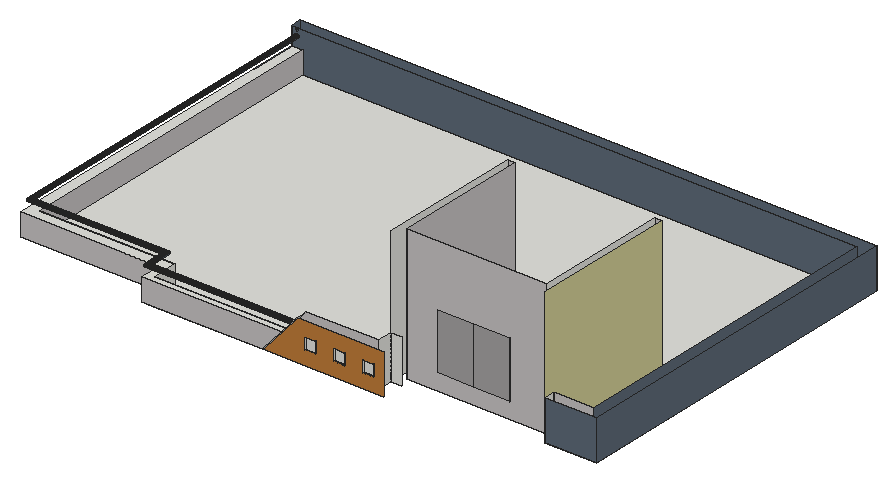
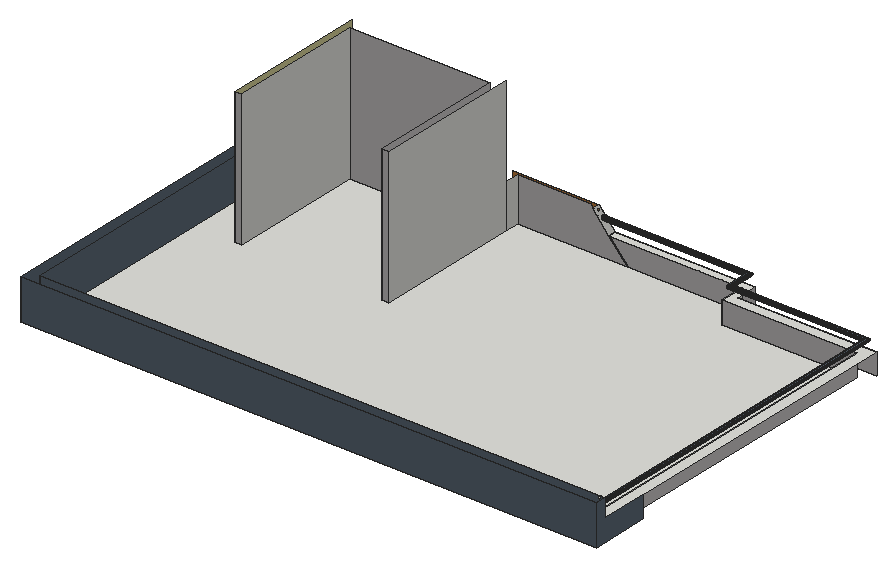
# SketchUp Ruby script. Lengths in inches.
U = 1.inch
M = Sketchup.active_model
def pt(a) = Geom::Point3d.new(a.map { |v| v * U })
def face(e, loops, mat)
  f = e.add_face(loops[0].map { |a| pt(a) })
  loops[1..].each { |l| e.add_face(l.map { |a| pt(a) }).erase! }
  f.material = f.back_material = mat if mat
  f
end
# faces: each face lists its corners as indices into pts; further lists are holes
def faces(e, pts, list, mat = nil) = list.each { |f| face(e, (f[0].is_a?(Array) ? f : [f]).map { |l| l.map { |i| pts[i] } }, mat) }
# xy, xz, yz: faces in a plane at the given z, y or x. An outline is a flat list of corners, or four numbers for a rectangle; further outlines are holes
def ring(l) = l.size == 4 ? [[l[0], l[1]], [l[2], l[1]], [l[2], l[3]], [l[0], l[3]]] : l.each_slice(2).to_a
def flat(e, list, mat, &to3) = list.each { |f| face(e, (f[0].is_a?(Array) ? f : [f]).map { |l| ring(l).map { |u, v| to3.(u, v) } }, mat) }
def xy(e, z, list, mat = nil) = flat(e, list, mat) { |x, y| [x, y, z] }
def xz(e, y, list, mat = nil) = flat(e, list, mat) { |x, z| [x, y, z] }
def yz(e, x, list, mat = nil) = flat(e, list, mat) { |y, z| [x, y, z] }
def lines(e, pts, list) = list.each { |a, b| e.add_line(pt(pts[a]), pt(pts[b])) }
# prism: a flat outline (further loops are holes) pulled along v
def prism(e, loops, v, mat = nil)
  f = face(e, loops, mat); d = Geom::Vector3d.new(v.map { |x| x * U })
  f.pushpull(f.normal.samedirection?(d) ? d.length : -d.length)
end
def box(e, o, s, mat = nil) = prism(e, [[o, [o[0] + s[0], o[1], o[2]], [o[0] + s[0], o[1] + s[1], o[2]], [o[0], o[1] + s[1], o[2]]]], [0, 0, s[2]], mat)
def at(x, y, z, deg = 0) = Geom::Transformation.translation(pt([x, y, z])) * Geom::Transformation.rotation(ORIGIN, Z_AXIS, deg.degrees)
def axes(o, x, y, z) = Geom::Transformation.new([*x, 0, *y, 0, *z, 0, *pt(o).to_a, 1])
def part(name) = M.definitions.add(name)
# library, detail: a bought-in or finely detailed component or shape, given as its bounding box
def library(name, o, s) = part(name).tap { |d| box(d.entities, o, s) }
def detail(e, o, s) = box(e.add_group.entities, o, s)
def put(e, d, t, mat = nil) = e.add_instance(d, t).tap { |i| i.material = mat if mat }
def group(e, t, mat = nil) = e.add_group.tap { |g| g.transformation = t; g.material = mat if mat }.entities
root = M.entities
M.materials.add("[0010_Snow]").color = [198, 195, 195]
M.materials.add("[0040_Peru]").color = [191, 124, 58]
M.materials.add("[0048_PaleGoldenrod]").color = [211, 206, 151]
M.materials.add("[0111_SlateGray]").color = [93, 106, 119]
M.materials.add("[Translucent Glass Gray]").color = [128, 128, 128]
M.materials["[Translucent Glass Gray]"].alpha = 0.5
xy(root,660,[[240,27,427.91,39],[240,39,609.8125,39,609.8125,303,621.8125,303,621.8125,81,852,81,852,303,864,303,864,81,930,81,930,621,18,621,18,81,240,81],[864,63,864,81,930,81,930,621,0,621,0,639,948,639,948,63]])
xy(root,683.75,[[496.66,27,515.34,29],[544.66,27,563.34,29],[592.66,27,611.34,29]])
xy(root,696,[[228,27,458.85,27,458.85,39,240,39,240,81,18,81,18,621,0,621,0,63,228,63]])
xy(root,702.43,[[496.66,27,515.34,29],[544.66,27,563.34,29],[592.66,27,611.34,29]])
xz(root,27,[[228,660,427.91,660,458.85,696,228,696]],"[0010_Snow]")
xz(root,27,[[[427.91,660,627.8125,660,627.8125,726.875,485.39,726.875,458.85,696],[544.66,683.75,563.34,702.43],[496.66,683.75,515.34,702.43],[592.66,683.75,611.34,702.43]]],"[0040_Peru]")
xz(root,29,[[496.66,683.75,515.34,702.43],[544.66,683.75,563.34,702.43],[592.66,683.75,611.34,702.43]])
xz(root,39,[[240,660,240,696,458.85,696,427.91,660],[427.91,660,458.85,696,485.39,726.875,489.79,732,609.8125,732,609.8125,660]],"[0010_Snow]")
xz(root,63,[[609.8125,660,627.8125,732]])
xz(root,63,[[0,660,228,696]],"[0010_Snow]")
xz(root,63,[[864,660,948,726]],"[0111_SlateGray]")
xz(root,63,[[687,699.72,746.59,793.97],[746.59,699.72,806.18,793.97]],"[Translucent Glass Gray]")
xz(root,81,[[18,660,240,696],[621.8125,660,852,882],[864,660,930,726]],"[0010_Snow]")
xz(root,303,[[609.8125,660,621.8125,882],[852,660,864,882]],"[0010_Snow]")
xz(root,621,[[9,711,8.6875,711.02,8.375,711.07,8.07,711.15,7.78,711.26,7.5,711.4,7.24,711.57,6.99,711.77,6.77,711.99,6.57,712.24,6.4,712.5,6.26,712.78,6.15,713.07,6.07,713.375,6.02,713.6875,6,714,6.02,714.3125,6.07,714.625,6.15,714.93,6.26,715.22,6.4,715.5,6.57,715.76,6.77,716.01,6.99,716.23,7.24,716.43,7.5,716.6,7.78,716.74,8.07,716.85,8.375,716.93,8.6875,716.98,9,717,9.3125,716.98,9.625,716.93,9.93,716.85,10.22,716.74,10.5,716.6,10.76,716.43,11.01,716.23,11.23,716.01,11.43,715.76,11.6,715.5,11.74,715.22,11.85,714.93,11.93,714.625,11.98,714.3125,12,714,11.98,713.6875,11.93,713.375,11.85,713.07,11.74,712.78,11.6,712.5,11.43,712.24,11.23,711.99,11.01,711.77,10.76,711.57,10.5,711.4,10.22,711.26,9.93,711.15,9.625,711.07,9.3125,711.02]])
xz(root,621,[[[18,660,930,660,930,726,0,726,0,696,18,696],[9,711,8.6875,711.02,8.375,711.07,8.07,711.15,7.78,711.26,7.5,711.4,7.24,711.57,6.99,711.77,6.77,711.99,6.57,712.24,6.4,712.5,6.26,712.78,6.15,713.07,6.07,713.375,6.02,713.6875,6,714,6.02,714.3125,6.07,714.625,6.15,714.93,6.26,715.22,6.4,715.5,6.57,715.76,6.77,716.01,6.99,716.23,7.24,716.43,7.5,716.6,7.78,716.74,8.07,716.85,8.375,716.93,8.6875,716.98,9,717,9.3125,716.98,9.625,716.93,9.93,716.85,10.22,716.74,10.5,716.6,10.76,716.43,11.01,716.23,11.23,716.01,11.43,715.76,11.6,715.5,11.74,715.22,11.85,714.93,11.93,714.625,11.98,714.3125,12,714,11.98,713.6875,11.93,713.375,11.85,713.07,11.74,712.78,11.6,712.5,11.43,712.24,11.23,711.99,11.01,711.77,10.76,711.57,10.5,711.4,10.22,711.26,9.93,711.15,9.625,711.07,9.3125,711.02],[9,720,8.6875,720.02,8.375,720.07,8.07,720.15,7.78,720.26,7.5,720.4,7.24,720.57,6.99,720.77,6.77,720.99,6.57,721.24,6.4,721.5,6.26,721.78,6.15,722.07,6.07,722.375,6.02,722.6875,6,723,6.02,723.3125,6.07,723.625,6.15,723.93,6.26,724.22,6.4,724.5,6.57,724.76,6.77,725.01,6.99,725.23,7.24,725.43,7.5,725.6,7.78,725.74,8.07,725.85,8.375,725.93,8.6875,725.98,9,726,9.3125,725.98,9.625,725.93,9.93,725.85,10.22,725.74,10.5,725.6,10.76,725.43,11.01,725.23,11.23,725.01,11.43,724.76,11.6,724.5,11.74,724.22,11.85,723.93,11.93,723.625,11.98,723.3125,12,723,11.98,722.6875,11.93,722.375,11.85,722.07,11.74,721.78,11.6,721.5,11.43,721.24,11.23,720.99,11.01,720.77,10.76,720.57,10.5,720.4,10.22,720.26,9.93,720.15,9.625,720.07,9.3125,720.02]]],"[0111_SlateGray]")
xz(root,639,[[0,660,948,726]],"[0111_SlateGray]")
yz(root,0,[[543,660,543,696,621,696,621,726,639,726,639,660]],"[0111_SlateGray]")
yz(root,18,[[81,660,621,696]],"[0010_Snow]")
yz(root,240,[[39,660,81,696]])
yz(root,474.32,[[32,711,32.3125,711.02,32.625,711.07,32.93,711.15,33.22,711.26,33.5,711.4,33.76,711.57,34.01,711.77,34.23,711.99,34.43,712.24,34.6,712.5,34.74,712.78,34.85,713.07,34.93,713.375,34.98,713.6875,35,714,34.98,714.3125,34.93,714.625,34.85,714.93,34.74,715.22,34.6,715.5,34.43,715.76,34.23,716.01,34.01,716.23,33.76,716.43,33.5,716.6,33.22,716.74,32.93,716.85,32.625,716.93,32.3125,716.98,32,717,31.6875,716.98,31.375,716.93,31.07,716.85,30.78,716.74,30.5,716.6,30.24,716.43,29.99,716.23,29.77,716.01,29.57,715.76,29.4,715.5,29.26,715.22,29.15,714.93,29.07,714.625,29.02,714.3125,29,714,29.02,713.6875,29.07,713.375,29.15,713.07,29.26,712.78,29.4,712.5,29.57,712.24,29.77,711.99,29.99,711.77,30.24,711.57,30.5,711.4,30.78,711.26,31.07,711.15,31.375,711.07,31.6875,711.02]])
yz(root,496.66,[[27,683.75,29,702.43]])
yz(root,515.34,[[27,683.75,29,702.43]])
yz(root,544.66,[[27,683.75,29,702.43]])
yz(root,563.34,[[27,683.75,29,702.43]])
yz(root,592.66,[[27,683.75,29,702.43]])
yz(root,609.8125,[[39,660,63,732],[63,660,303,882]])
yz(root,611.34,[[27,683.75,29,702.43]])
yz(root,621.8125,[[81,660,303,882]],"[0010_Snow]")
yz(root,806.18,[[62,699.72,63,793.97]])
yz(root,852,[[81,660,303,882]])
yz(root,864,[[63,660,81,726]])
yz(root,864,[[81,660,303,660,303,882,63,882,63,726,81,726]],"[0048_PaleGoldenrod]")
yz(root,930,[[81,660,621,726]],"[0111_SlateGray]")
yz(root,948,[[63,660,639,726]],"[0111_SlateGray]")
p = [[427.91,27,660],[458.85,27,696],[458.85,39,696],[427.91,39,660],[485.39,39,726.875],[485.39,27,726.875],
  [483.86,33.16,725.1],[483.93,32.87,725.18],[483.98,32.5625,725.23],[484,32.25,725.27],[484.01,31.94,725.27],[484,31.625,725.26],
  [483.96,31.32,725.22],[483.9,31.02,725.15],[483.83,30.72,725.06],[483.73,30.45,724.95],[483.61,30.1875,724.8125],[483.48,29.95,724.66],
  [483.33,29.73,724.49],[483.17,29.54,724.3],[483,29.37,724.1],[482.8125,29.24,723.88],[482.62,29.13,723.66],[482.42,29.05,723.43],
  [482.22,29.01,723.19],[482.02,29,722.95],[481.8125,29.02,722.72],[481.61,29.08,722.48],[481.41,29.17,722.25],[481.22,29.28,722.03],
  [481.04,29.43,721.82],[480.875,29.61,721.625],[480.72,29.8125,721.44],[480.58,30.04,721.28],[480.45,30.29,721.13],[480.34,30.55,721.01],
  [480.25,30.84,720.9],[480.18,31.13,720.82],[480.13,31.4375,720.77],[480.11,31.75,720.73],[480.1,32.06,720.73],[480.11,32.375,720.74],
  [480.15,32.68,720.78],[480.21,32.98,720.85],[480.29,33.28,720.94],[480.38,33.55,721.05],[480.5,33.8125,721.1875],[480.63,34.05,721.34],
  [480.78,34.27,721.51],[480.9375,34.46,721.7],[481.11,34.63,721.9],[481.3,34.76,722.12],[481.49,34.87,722.34],[481.6875,34.95,722.57],
  [481.89,34.99,722.81],[482.09,35,723.05],[482.3,34.98,723.28],[482.5,34.92,723.52],[482.7,34.83,723.75],[482.89,34.72,723.97],
  [483.07,34.57,724.18],[483.24,34.39,724.375],[483.39,34.1875,724.56],[483.53,33.96,724.72],[483.66,33.71,724.87],[483.77,33.45,724.99],
  [476.21,31.22,716.2],[476.01,30.5,715.97],[475.7,29.88,715.61],[475.3,29.4,715.14],[474.83,29.1,714.59],[474.32,29,714],
  [473.8125,29.1,713.41],[473.34,29.4,712.86],[472.9375,29.88,712.39],[472.625,30.5,712.03],[472.43,31.22,711.8],[472.36,32,711.72],
  [472.43,32.78,711.8],[472.625,33.5,712.03],[472.9375,34.12,712.39],[473.34,34.6,712.86],[473.8125,34.9,713.41],[474.32,35,714],
  [474.83,34.9,714.59],[475.3,34.6,715.14],[475.7,34.12,715.61],[476.01,33.5,715.97],[476.21,32.78,716.2],[476.28,32,716.28],
  [233.375,71.375,711.07],[233.6875,71.6875,711.02],[233.6875,31.6875,711.02],[233.375,31.375,711.07],[474.32,31.6875,711.02],[474.32,31.375,711.07],
  [234,72,711],[234,32,711],[474.32,32,711],[234.3125,72.3125,711.02],[234.3125,32.3125,711.02],[474.32,32.3125,711.02],
  [234.625,72.625,711.07],[234.625,32.625,711.07],[474.32,32.625,711.07],[8.375,621,711.07],[8.6875,621,711.02],[8.6875,71.6875,711.02],
  [8.375,71.375,711.07],[9,621,711],[9,72,711],[9.3125,621,711.02],[9.3125,72.3125,711.02],[9.625,621,711.07],
  [9.625,72.625,711.07],[232.78,70.78,711.26],[233.07,71.07,711.15],[233.07,31.07,711.15],[232.78,30.78,711.26],[474.32,31.07,711.15],
  [474.32,30.78,711.26],[234.93,72.93,711.15],[234.93,32.93,711.15],[474.32,32.93,711.15],[235.22,73.22,711.26],[235.22,33.22,711.26],
  [474.32,33.22,711.26],[7.78,621,711.26],[8.07,621,711.15],[8.07,71.07,711.15],[7.78,70.78,711.26],[9.93,621,711.15],
  [9.93,72.93,711.15],[10.22,621,711.26],[10.22,73.22,711.26],[232.5,70.5,711.4],[232.5,30.5,711.4],[474.32,30.5,711.4],
  [235.5,73.5,711.4],[235.5,33.5,711.4],[474.32,33.5,711.4],[7.5,621,711.4],[7.5,70.5,711.4],[10.5,621,711.4],
  [10.5,73.5,711.4],[232.24,70.24,711.57],[232.24,30.24,711.57],[474.32,30.24,711.57],[235.76,73.76,711.57],[235.76,33.76,711.57],
  [474.32,33.76,711.57],[7.24,621,711.57],[7.24,70.24,711.57],[10.76,621,711.57],[10.76,73.76,711.57],[231.99,69.99,711.77],
  [231.99,29.99,711.77],[474.32,29.99,711.77],[236.01,74.01,711.77],[236.01,34.01,711.77],[474.32,34.01,711.77],[6.99,621,711.77],
  [6.99,69.99,711.77],[11.01,621,711.77],[11.01,74.01,711.77],[231.77,69.77,711.99],[231.77,29.77,711.99],[474.32,29.77,711.99],
  [236.23,74.23,711.99],[236.23,34.23,711.99],[474.32,34.23,711.99],[6.77,621,711.99],[6.77,69.77,711.99],[11.23,621,711.99],
  [11.23,74.23,711.99],[231.57,69.57,712.24],[231.57,29.57,712.24],[474.32,29.57,712.24],[236.43,74.43,712.24],[236.43,34.43,712.24],
  [474.32,34.43,712.24],[6.57,621,712.24],[6.57,69.57,712.24],[11.43,621,712.24],[11.43,74.43,712.24],[231.4,69.4,712.5],
  [231.4,29.4,712.5],[474.32,29.4,712.5],[236.6,74.6,712.5],[236.6,34.6,712.5],[474.32,34.6,712.5],[6.4,621,712.5],
  [6.4,69.4,712.5],[11.6,621,712.5],[11.6,74.6,712.5],[231.26,69.26,712.78],[231.26,29.26,712.78],[474.32,29.26,712.78],
  [236.74,74.74,712.78],[236.74,34.74,712.78],[474.32,34.74,712.78],[6.26,621,712.78],[6.26,69.26,712.78],[11.74,621,712.78],
  [11.74,74.74,712.78],[231.15,69.15,713.07],[231.15,29.15,713.07],[474.32,29.15,713.07],[236.85,74.85,713.07],[236.85,34.85,713.07],
  [474.32,34.85,713.07],[6.15,621,713.07],[6.15,69.15,713.07],[11.85,621,713.07],[11.85,74.85,713.07],[231.07,69.07,713.375],
  [231.07,29.07,713.375],[474.32,29.07,713.375],[236.93,74.93,713.375],[236.93,34.93,713.375],[474.32,34.93,713.375],[6.07,621,713.375],
  [6.07,69.07,713.375],[11.93,621,713.375],[11.93,74.93,713.375],[231.02,69.02,713.6875],[231.02,29.02,713.6875],[474.32,29.02,713.6875],
  [236.98,74.98,713.6875],[236.98,34.98,713.6875],[474.32,34.98,713.6875],[6.02,621,713.6875],[6.02,69.02,713.6875],[11.98,621,713.6875],
  [11.98,74.98,713.6875],[231,69,714],[231,29,714],[237,75,714],[237,35,714],[6,621,714],
  [6,69,714],[12,621,714],[12,75,714],[231.02,69.02,714.3125],[231.02,29.02,714.3125],[474.32,29.02,714.3125],
  [236.98,74.98,714.3125],[236.98,34.98,714.3125],[474.32,34.98,714.3125],[6.02,621,714.3125],[6.02,69.02,714.3125],[11.98,621,714.3125],
  [11.98,74.98,714.3125],[231.07,69.07,714.625],[231.07,29.07,714.625],[474.32,29.07,714.625],[236.93,74.93,714.625],[236.93,34.93,714.625],
  [474.32,34.93,714.625],[6.07,621,714.625],[6.07,69.07,714.625],[11.93,621,714.625],[11.93,74.93,714.625],[231.15,69.15,714.93],
  [231.15,29.15,714.93],[474.32,29.15,714.93],[236.85,74.85,714.93],[236.85,34.85,714.93],[474.32,34.85,714.93],[6.15,621,714.93],
  [6.15,69.15,714.93],[11.85,621,714.93],[11.85,74.85,714.93],[231.26,69.26,715.22],[231.26,29.26,715.22],[474.32,29.26,715.22],
  [236.74,74.74,715.22],[236.74,34.74,715.22],[474.32,34.74,715.22],[6.26,621,715.22],[6.26,69.26,715.22],[11.74,621,715.22],
  [11.74,74.74,715.22],[231.4,69.4,715.5],[231.4,29.4,715.5],[474.32,29.4,715.5],[236.6,74.6,715.5],[236.6,34.6,715.5],
  [474.32,34.6,715.5],[6.4,621,715.5],[6.4,69.4,715.5],[11.6,621,715.5],[11.6,74.6,715.5],[231.57,69.57,715.76],
  [231.57,29.57,715.76],[474.32,29.57,715.76],[236.43,74.43,715.76],[236.43,34.43,715.76],[474.32,34.43,715.76],[6.57,621,715.76],
  [6.57,69.57,715.76],[11.43,621,715.76],[11.43,74.43,715.76],[231.77,69.77,716.01],[231.77,29.77,716.01],[474.32,29.77,716.01],
  [236.23,74.23,716.01],[236.23,34.23,716.01],[474.32,34.23,716.01],[6.77,621,716.01],[6.77,69.77,716.01],[11.23,621,716.01],
  [11.23,74.23,716.01],[231.99,69.99,716.23],[231.99,29.99,716.23],[474.32,29.99,716.23],[236.01,74.01,716.23],[236.01,34.01,716.23],
  [474.32,34.01,716.23],[6.99,621,716.23],[6.99,69.99,716.23],[11.01,621,716.23],[11.01,74.01,716.23],[232.24,70.24,716.43],
  [232.24,30.24,716.43],[474.32,30.24,716.43],[235.76,73.76,716.43],[235.76,33.76,716.43],[474.32,33.76,716.43],[7.24,621,716.43],
  [7.24,70.24,716.43],[10.76,621,716.43],[10.76,73.76,716.43],[232.5,70.5,716.6],[232.5,30.5,716.6],[474.32,30.5,716.6],
  [235.5,73.5,716.6],[235.5,33.5,716.6],[474.32,33.5,716.6],[7.5,621,716.6],[7.5,70.5,716.6],[10.5,621,716.6],
  [10.5,73.5,716.6],[232.78,70.78,716.74],[232.78,30.78,716.74],[474.32,30.78,716.74],[235.22,73.22,716.74],[235.22,33.22,716.74],
  [474.32,33.22,716.74],[7.78,621,716.74],[7.78,70.78,716.74],[10.22,621,716.74],[10.22,73.22,716.74],[233.07,71.07,716.85],
  [233.07,31.07,716.85],[474.32,31.07,716.85],[234.93,72.93,716.85],[234.93,32.93,716.85],[474.32,32.93,716.85],[8.07,621,716.85],
  [8.07,71.07,716.85],[9.93,621,716.85],[9.93,72.93,716.85],[233.375,71.375,716.93],[233.375,31.375,716.93],[474.32,31.375,716.93],
  [233.6875,71.6875,716.98],[233.6875,31.6875,716.98],[474.32,31.6875,716.98],[234.625,72.625,716.93],[234.3125,72.3125,716.98],[234.3125,32.3125,716.98],
  [234.625,32.625,716.93],[474.32,32.3125,716.98],[474.32,32.625,716.93],[8.375,621,716.93],[8.375,71.375,716.93],[8.6875,621,716.98],
  [8.6875,71.6875,716.98],[9.625,621,716.93],[9.3125,621,716.98],[9.3125,72.3125,716.98],[9.625,72.625,716.93],[234,72,717],
  [234,32,717],[474.32,32,717],[9,621,717],[9,72,717],[234,32,714],[474.32,32,714],
  [234,72,714],[9,72,714],[9,621,714]]
faces(root,p,[[0,1,2,3],[[4,2,1,5],[6,7,8,9,10,11,12,13,14,15,16,17,18,19,20,21,22,23,24,25,26,27,28,29,30,31,32,33,34,35,36,37,38,39,40,41,42,43,44,45,46,47,48,49,50,51,52,53,54,55,56,57,58,59,60,61,62,63,64,65],[66,67,68,69,70,71,72,73,74,75,76,77,78,79,80,81,82,83,84,85,86,87,88,89]],[67,66,89,88,87,86,85,84,83,82,81,80,79,78,77,76,75,74,73,72,71,70,69,68]])
faces(root,p,[[90,91,92,93],[93,92,94,95],[91,96,97,92],[92,97,98,94],[96,99,100,97],[97,100,101,98],[99,102,103,100],[100,103,104,101],
  [105,106,107,108],[108,107,91,90],[106,109,110,107],[107,110,96,91],[109,111,112,110],[110,112,99,96],[111,113,114,112],[112,114,102,99],
  [115,116,117,118],[118,117,119,120],[116,90,93,117],[117,93,95,119],[102,121,122,103],[103,122,123,104],[121,124,125,122],[122,125,126,123],
  [127,128,129,130],[130,129,116,115],[128,105,108,129],[129,108,90,116],[113,131,132,114],[114,132,121,102],[131,133,134,132],[132,134,124,121],
  [135,115,118,136],[136,118,120,137],[124,138,139,125],[125,139,140,126],[141,127,130,142],[142,130,115,135],[133,143,144,134],[134,144,138,124],
  [145,135,136,146],[146,136,137,147],[138,148,149,139],[139,149,150,140],[151,141,142,152],[152,142,135,145],[143,153,154,144],[144,154,148,138],
  [155,145,146,156],[156,146,147,157],[148,158,159,149],[149,159,160,150],[161,151,152,162],[162,152,145,155],[153,163,164,154],[154,164,158,148],
  [165,155,156,166],[166,156,157,167],[158,168,169,159],[159,169,170,160],[171,161,162,172],[172,162,155,165],[163,173,174,164],[164,174,168,158],
  [175,165,166,176],[176,166,167,177],[168,178,179,169],[169,179,180,170],[181,171,172,182],[182,172,165,175],[173,183,184,174],[174,184,178,168],
  [185,175,176,186],[186,176,177,187],[178,188,189,179],[179,189,190,180],[191,181,182,192],[192,182,175,185],[183,193,194,184],[184,194,188,178],
  [195,185,186,196],[196,186,187,197],[188,198,199,189],[189,199,200,190],[201,191,192,202],[202,192,185,195],[193,203,204,194],[194,204,198,188],
  [205,195,196,206],[206,196,197,207],[198,208,209,199],[199,209,210,200],[211,201,202,212],[212,202,195,205],[203,213,214,204],[204,214,208,198],
  [215,205,206,216],[216,206,207,217],[208,218,219,209],[209,219,220,210],[221,211,212,222],[222,212,205,215],[213,223,224,214],[214,224,218,208],
  [225,215,216,226],[226,216,217,227],[218,228,229,219],[219,229,230,220],[231,221,222,232],[232,222,215,225],[223,233,234,224],[224,234,228,218],
  [235,225,226,236],[236,226,227,71],[228,237,238,229],[229,238,83,230],[239,231,232,240],[240,232,225,235],[233,241,242,234],[234,242,237,228],
  [243,235,236,244],[244,236,71,245],[237,246,247,238],[238,247,248,83],[249,239,240,250],[250,240,235,243],[241,251,252,242],[242,252,246,237],
  [253,243,244,254],[254,244,245,255],[246,256,257,247],[247,257,258,248],[259,249,250,260],[260,250,243,253],[251,261,262,252],[252,262,256,246],
  [263,253,254,264],[264,254,255,265],[256,266,267,257],[257,267,268,258],[269,259,260,270],[270,260,253,263],[261,271,272,262],[262,272,266,256],
  [273,263,264,274],[274,264,265,275],[266,276,277,267],[267,277,278,268],[279,269,270,280],[280,270,263,273],[271,281,282,272],[272,282,276,266],
  [283,273,274,284],[284,274,275,285],[276,286,287,277],[277,287,288,278],[289,279,280,290],[290,280,273,283],[281,291,292,282],[282,292,286,276],
  [293,283,284,294],[294,284,285,295],[286,296,297,287],[287,297,298,288],[299,289,290,300],[300,290,283,293],[291,301,302,292],[292,302,296,286],
  [303,293,294,304],[304,294,295,305],[296,306,307,297],[297,307,308,298],[309,299,300,310],[310,300,293,303],[301,311,312,302],[302,312,306,296],
  [313,303,304,314],[314,304,305,315],[306,316,317,307],[307,317,318,308],[319,309,310,320],[320,310,303,313],[311,321,322,312],[312,322,316,306],
  [323,313,314,324],[324,314,315,325],[316,326,327,317],[317,327,328,318],[329,319,320,330],[330,320,313,323],[321,331,332,322],[322,332,326,316],
  [333,323,324,334],[334,324,325,335],[326,336,337,327],[327,337,338,328],[339,329,330,340],[340,330,323,333],[331,341,342,332],[332,342,336,326],
  [343,333,334,344],[344,334,335,345],[336,346,347,337],[337,347,348,338],[349,339,340,350],[350,340,333,343],[341,351,352,342],[342,352,346,336],
  [353,343,344,354],[354,344,345,355],[346,356,357,347],[347,357,358,348],[359,349,350,360],[360,350,343,353],[351,361,362,352],[352,362,356,346],
  [363,353,354,364],[364,354,355,365],[366,363,364,367],[367,364,365,368],[369,370,371,372],[372,371,373,374],[356,369,372,357],[357,372,374,358],
  [375,359,360,376],[376,360,353,363],[377,375,376,378],[378,376,363,366],[379,380,381,382],[382,381,370,369],[361,379,382,362],[362,382,369,356],
  [383,366,367,384],[384,367,368,385],[370,383,384,371],[371,384,385,373],[386,377,378,387],[387,378,366,383],[380,386,387,381],[381,387,383,370]],"[0111_SlateGray]")
lines(root,p,[[388,384],[388,389],[390,383],[388,390],[390,391],[391,392],[97,388],[96,390],[110,391],[391,387]])
